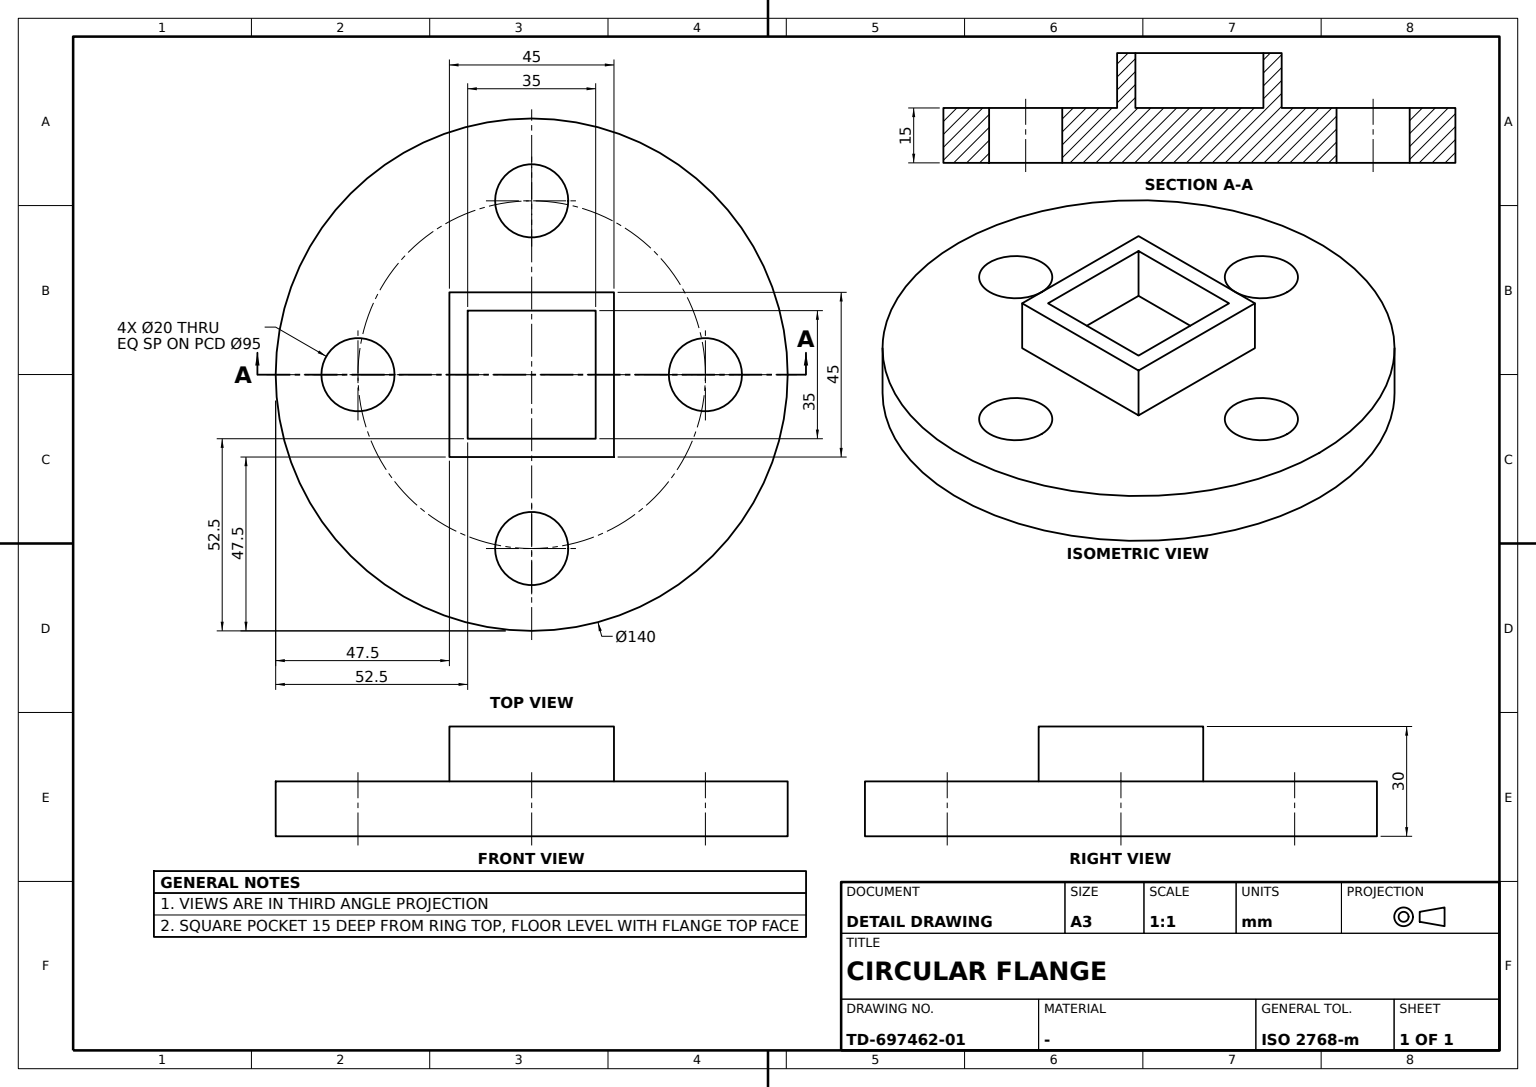
ISO-10303-21;
HEADER;
FILE_DESCRIPTION((''),'2;1');
FILE_NAME('','',(''),(''),'','','');
FILE_SCHEMA(('AUTOMOTIVE_DESIGN'));
ENDSEC;
DATA;
#1=APPLICATION_CONTEXT('');
#2=PRODUCT_CONTEXT('',#1,'mechanical');
#3=PRODUCT('','','',(#2));
#4=PRODUCT_DEFINITION_FORMATION('','',#3);
#5=PRODUCT_DEFINITION_CONTEXT('',#1,'design');
#6=PRODUCT_DEFINITION('','',#4,#5);
#7=PRODUCT_DEFINITION_SHAPE('','',#6);
#8=(LENGTH_UNIT()NAMED_UNIT(*)SI_UNIT(.MILLI.,.METRE.));
#9=(NAMED_UNIT(*)PLANE_ANGLE_UNIT()SI_UNIT($,.RADIAN.));
#10=(NAMED_UNIT(*)SI_UNIT($,.STERADIAN.)SOLID_ANGLE_UNIT());
#11=UNCERTAINTY_MEASURE_WITH_UNIT(LENGTH_MEASURE(0.005),#8,'distance_accuracy_value','');
#12=(GEOMETRIC_REPRESENTATION_CONTEXT(3)GLOBAL_UNCERTAINTY_ASSIGNED_CONTEXT((#11))GLOBAL_UNIT_ASSIGNED_CONTEXT((#8,#9,#10))REPRESENTATION_CONTEXT('',''));
#13=CARTESIAN_POINT('',(-17.5,-17.5,15.));
#14=VERTEX_POINT('',#13);
#15=CARTESIAN_POINT('',(-17.5,17.5,15.));
#16=VERTEX_POINT('',#15);
#17=CARTESIAN_POINT('',(-17.5,0.,15.));
#18=DIRECTION('',(0.,1.,0.));
#19=VECTOR('',#18,1000.);
#20=LINE('',#17,#19);
#21=EDGE_CURVE('',#14,#16,#20,.T.);
#22=ORIENTED_EDGE('',*,*,#21,.F.);
#23=CARTESIAN_POINT('',(17.5,-17.5,15.));
#24=VERTEX_POINT('',#23);
#25=CARTESIAN_POINT('',(0.,-17.5,15.));
#26=DIRECTION('',(-1.,0.,0.));
#27=VECTOR('',#26,1000.);
#28=LINE('',#25,#27);
#29=EDGE_CURVE('',#24,#14,#28,.T.);
#30=ORIENTED_EDGE('',*,*,#29,.F.);
#31=CARTESIAN_POINT('',(17.5,17.5,15.));
#32=VERTEX_POINT('',#31);
#33=CARTESIAN_POINT('',(17.5,0.,15.));
#34=DIRECTION('',(0.,-1.,0.));
#35=VECTOR('',#34,1000.);
#36=LINE('',#33,#35);
#37=EDGE_CURVE('',#32,#24,#36,.T.);
#38=ORIENTED_EDGE('',*,*,#37,.F.);
#39=CARTESIAN_POINT('',(0.,17.5,15.));
#40=DIRECTION('',(1.,0.,0.));
#41=VECTOR('',#40,1000.);
#42=LINE('',#39,#41);
#43=EDGE_CURVE('',#16,#32,#42,.T.);
#44=ORIENTED_EDGE('',*,*,#43,.F.);
#45=EDGE_LOOP('',(#22,#30,#38,#44));
#46=FACE_BOUND('',#45,.T.);
#47=CARTESIAN_POINT('',(0.,0.,15.));
#48=DIRECTION('',(0.,0.,1.));
#49=AXIS2_PLACEMENT_3D('',#47,#48,#40);
#50=PLANE('',#49);
#51=ADVANCED_FACE('',(#46),#50,.T.);
#52=CARTESIAN_POINT('',(-22.5,22.5,15.));
#53=VERTEX_POINT('',#52);
#54=CARTESIAN_POINT('',(-22.5,22.5,30.));
#55=VERTEX_POINT('',#54);
#56=VECTOR('',#48,1000.);
#57=LINE('',#52,#56);
#58=EDGE_CURVE('',#53,#55,#57,.T.);
#59=ORIENTED_EDGE('',*,*,#58,.T.);
#60=CARTESIAN_POINT('',(22.5,22.5,30.));
#61=VERTEX_POINT('',#60);
#62=CARTESIAN_POINT('',(0.,22.5,30.));
#63=LINE('',#62,#41);
#64=EDGE_CURVE('',#55,#61,#63,.T.);
#65=ORIENTED_EDGE('',*,*,#64,.T.);
#66=CARTESIAN_POINT('',(22.5,22.5,15.));
#67=VERTEX_POINT('',#66);
#68=LINE('',#66,#56);
#69=EDGE_CURVE('',#67,#61,#68,.T.);
#70=ORIENTED_EDGE('',*,*,#69,.F.);
#71=CARTESIAN_POINT('',(0.,22.5,15.));
#72=LINE('',#71,#41);
#73=EDGE_CURVE('',#53,#67,#72,.T.);
#74=ORIENTED_EDGE('',*,*,#73,.F.);
#75=EDGE_LOOP('',(#59,#65,#70,#74));
#76=FACE_BOUND('',#75,.T.);
#77=AXIS2_PLACEMENT_3D('',#52,#34,#40);
#78=PLANE('',#77);
#79=ADVANCED_FACE('',(#76),#78,.F.);
#80=CARTESIAN_POINT('',(-37.5,0.,0.));
#81=VERTEX_POINT('',#80);
#82=CARTESIAN_POINT('',(-47.5,0.,0.));
#83=AXIS2_PLACEMENT_3D('',#82,#48,#40);
#84=CIRCLE('',#83,10.);
#85=EDGE_CURVE('',#81,#81,#84,.T.);
#86=ORIENTED_EDGE('',*,*,#85,.F.);
#87=EDGE_LOOP('',(#86));
#88=FACE_BOUND('',#87,.T.);
#89=CARTESIAN_POINT('',(-37.5,0.,15.));
#90=VERTEX_POINT('',#89);
#91=CARTESIAN_POINT('',(-47.5,0.,15.));
#92=AXIS2_PLACEMENT_3D('',#91,#48,#40);
#93=CIRCLE('',#92,10.);
#94=EDGE_CURVE('',#90,#90,#93,.T.);
#95=ORIENTED_EDGE('',*,*,#94,.T.);
#96=EDGE_LOOP('',(#95));
#97=FACE_BOUND('',#96,.T.);
#98=CARTESIAN_POINT('',(-47.5,0.,7.5));
#99=AXIS2_PLACEMENT_3D('',#98,#48,#40);
#100=CYLINDRICAL_SURFACE('',#99,10.);
#101=ADVANCED_FACE('',(#88,#97),#100,.F.);
#102=CARTESIAN_POINT('',(-17.5,17.5,30.));
#103=VERTEX_POINT('',#102);
#104=CARTESIAN_POINT('',(17.5,17.5,30.));
#105=VERTEX_POINT('',#104);
#106=CARTESIAN_POINT('',(0.,17.5,30.));
#107=LINE('',#106,#41);
#108=EDGE_CURVE('',#103,#105,#107,.T.);
#109=ORIENTED_EDGE('',*,*,#108,.T.);
#110=CARTESIAN_POINT('',(17.5,-17.5,30.));
#111=VERTEX_POINT('',#110);
#112=CARTESIAN_POINT('',(17.5,0.,30.));
#113=LINE('',#112,#35);
#114=EDGE_CURVE('',#105,#111,#113,.T.);
#115=ORIENTED_EDGE('',*,*,#114,.T.);
#116=CARTESIAN_POINT('',(-17.5,-17.5,30.));
#117=VERTEX_POINT('',#116);
#118=CARTESIAN_POINT('',(0.,-17.5,30.));
#119=LINE('',#118,#27);
#120=EDGE_CURVE('',#111,#117,#119,.T.);
#121=ORIENTED_EDGE('',*,*,#120,.T.);
#122=CARTESIAN_POINT('',(-17.5,0.,30.));
#123=LINE('',#122,#19);
#124=EDGE_CURVE('',#117,#103,#123,.T.);
#125=ORIENTED_EDGE('',*,*,#124,.T.);
#126=EDGE_LOOP('',(#109,#115,#121,#125));
#127=FACE_BOUND('',#126,.T.);
#128=CARTESIAN_POINT('',(22.5,-22.5,30.));
#129=VERTEX_POINT('',#128);
#130=CARTESIAN_POINT('',(-22.5,-22.5,30.));
#131=VERTEX_POINT('',#130);
#132=CARTESIAN_POINT('',(0.,-22.5,30.));
#133=LINE('',#132,#27);
#134=EDGE_CURVE('',#129,#131,#133,.T.);
#135=ORIENTED_EDGE('',*,*,#134,.F.);
#136=CARTESIAN_POINT('',(22.5,0.,30.));
#137=LINE('',#136,#35);
#138=EDGE_CURVE('',#61,#129,#137,.T.);
#139=ORIENTED_EDGE('',*,*,#138,.F.);
#140=ORIENTED_EDGE('',*,*,#64,.F.);
#141=CARTESIAN_POINT('',(-22.5,0.,30.));
#142=LINE('',#141,#19);
#143=EDGE_CURVE('',#131,#55,#142,.T.);
#144=ORIENTED_EDGE('',*,*,#143,.F.);
#145=EDGE_LOOP('',(#135,#139,#140,#144));
#146=FACE_BOUND('',#145,.T.);
#147=CARTESIAN_POINT('',(0.,0.,30.));
#148=AXIS2_PLACEMENT_3D('',#147,#48,#40);
#149=PLANE('',#148);
#150=ADVANCED_FACE('',(#127,#146),#149,.T.);
#151=CARTESIAN_POINT('',(70.,0.,15.));
#152=VERTEX_POINT('',#151);
#153=CIRCLE('',#49,70.);
#154=EDGE_CURVE('',#152,#152,#153,.T.);
#155=ORIENTED_EDGE('',*,*,#154,.T.);
#156=EDGE_LOOP('',(#155));
#157=FACE_BOUND('',#156,.T.);
#158=CARTESIAN_POINT('',(10.,-47.5,15.));
#159=VERTEX_POINT('',#158);
#160=CARTESIAN_POINT('',(0.,-47.5,15.));
#161=AXIS2_PLACEMENT_3D('',#160,#48,#40);
#162=CIRCLE('',#161,10.);
#163=EDGE_CURVE('',#159,#159,#162,.T.);
#164=ORIENTED_EDGE('',*,*,#163,.F.);
#165=EDGE_LOOP('',(#164));
#166=FACE_BOUND('',#165,.T.);
#167=ORIENTED_EDGE('',*,*,#73,.T.);
#168=CARTESIAN_POINT('',(22.5,-22.5,15.));
#169=VERTEX_POINT('',#168);
#170=CARTESIAN_POINT('',(22.5,0.,15.));
#171=LINE('',#170,#35);
#172=EDGE_CURVE('',#67,#169,#171,.T.);
#173=ORIENTED_EDGE('',*,*,#172,.T.);
#174=CARTESIAN_POINT('',(-22.5,-22.5,15.));
#175=VERTEX_POINT('',#174);
#176=CARTESIAN_POINT('',(0.,-22.5,15.));
#177=LINE('',#176,#27);
#178=EDGE_CURVE('',#169,#175,#177,.T.);
#179=ORIENTED_EDGE('',*,*,#178,.T.);
#180=CARTESIAN_POINT('',(-22.5,0.,15.));
#181=LINE('',#180,#19);
#182=EDGE_CURVE('',#175,#53,#181,.T.);
#183=ORIENTED_EDGE('',*,*,#182,.T.);
#184=EDGE_LOOP('',(#167,#173,#179,#183));
#185=FACE_BOUND('',#184,.T.);
#186=ORIENTED_EDGE('',*,*,#94,.F.);
#187=EDGE_LOOP('',(#186));
#188=FACE_BOUND('',#187,.T.);
#189=CARTESIAN_POINT('',(57.5,0.,15.));
#190=VERTEX_POINT('',#189);
#191=CARTESIAN_POINT('',(47.5,0.,15.));
#192=AXIS2_PLACEMENT_3D('',#191,#48,#40);
#193=CIRCLE('',#192,10.);
#194=EDGE_CURVE('',#190,#190,#193,.T.);
#195=ORIENTED_EDGE('',*,*,#194,.F.);
#196=EDGE_LOOP('',(#195));
#197=FACE_BOUND('',#196,.T.);
#198=CARTESIAN_POINT('',(10.,47.5,15.));
#199=VERTEX_POINT('',#198);
#200=CARTESIAN_POINT('',(0.,47.5,15.));
#201=AXIS2_PLACEMENT_3D('',#200,#48,#40);
#202=CIRCLE('',#201,10.);
#203=EDGE_CURVE('',#199,#199,#202,.T.);
#204=ORIENTED_EDGE('',*,*,#203,.F.);
#205=EDGE_LOOP('',(#204));
#206=FACE_BOUND('',#205,.T.);
#207=ADVANCED_FACE('',(#157,#166,#185,#188,#197,#206),#50,.T.);
#208=ORIENTED_EDGE('',*,*,#163,.T.);
#209=EDGE_LOOP('',(#208));
#210=FACE_BOUND('',#209,.T.);
#211=CARTESIAN_POINT('',(10.,-47.5,0.));
#212=VERTEX_POINT('',#211);
#213=CARTESIAN_POINT('',(0.,-47.5,0.));
#214=AXIS2_PLACEMENT_3D('',#213,#48,#40);
#215=CIRCLE('',#214,10.);
#216=EDGE_CURVE('',#212,#212,#215,.T.);
#217=ORIENTED_EDGE('',*,*,#216,.F.);
#218=EDGE_LOOP('',(#217));
#219=FACE_BOUND('',#218,.T.);
#220=CARTESIAN_POINT('',(0.,-47.5,7.5));
#221=AXIS2_PLACEMENT_3D('',#220,#48,#40);
#222=CYLINDRICAL_SURFACE('',#221,10.);
#223=ADVANCED_FACE('',(#210,#219),#222,.F.);
#224=LINE('',#174,#56);
#225=EDGE_CURVE('',#175,#131,#224,.T.);
#226=ORIENTED_EDGE('',*,*,#225,.T.);
#227=ORIENTED_EDGE('',*,*,#143,.T.);
#228=ORIENTED_EDGE('',*,*,#58,.F.);
#229=ORIENTED_EDGE('',*,*,#182,.F.);
#230=EDGE_LOOP('',(#226,#227,#228,#229));
#231=FACE_BOUND('',#230,.T.);
#232=AXIS2_PLACEMENT_3D('',#174,#40,#18);
#233=PLANE('',#232);
#234=ADVANCED_FACE('',(#231),#233,.F.);
#235=ORIENTED_EDGE('',*,*,#114,.F.);
#236=LINE('',#31,#56);
#237=EDGE_CURVE('',#32,#105,#236,.T.);
#238=ORIENTED_EDGE('',*,*,#237,.F.);
#239=ORIENTED_EDGE('',*,*,#37,.T.);
#240=LINE('',#23,#56);
#241=EDGE_CURVE('',#24,#111,#240,.T.);
#242=ORIENTED_EDGE('',*,*,#241,.T.);
#243=EDGE_LOOP('',(#235,#238,#239,#242));
#244=FACE_BOUND('',#243,.T.);
#245=AXIS2_PLACEMENT_3D('',#31,#26,#34);
#246=PLANE('',#245);
#247=ADVANCED_FACE('',(#244),#246,.T.);
#248=CARTESIAN_POINT('',(10.,47.5,0.));
#249=VERTEX_POINT('',#248);
#250=CARTESIAN_POINT('',(0.,47.5,0.));
#251=AXIS2_PLACEMENT_3D('',#250,#48,#40);
#252=CIRCLE('',#251,10.);
#253=EDGE_CURVE('',#249,#249,#252,.T.);
#254=ORIENTED_EDGE('',*,*,#253,.F.);
#255=EDGE_LOOP('',(#254));
#256=FACE_BOUND('',#255,.T.);
#257=ORIENTED_EDGE('',*,*,#203,.T.);
#258=EDGE_LOOP('',(#257));
#259=FACE_BOUND('',#258,.T.);
#260=CARTESIAN_POINT('',(0.,47.5,7.5));
#261=AXIS2_PLACEMENT_3D('',#260,#48,#40);
#262=CYLINDRICAL_SURFACE('',#261,10.);
#263=ADVANCED_FACE('',(#256,#259),#262,.F.);
#264=ORIENTED_EDGE('',*,*,#194,.T.);
#265=EDGE_LOOP('',(#264));
#266=FACE_BOUND('',#265,.T.);
#267=CARTESIAN_POINT('',(57.5,0.,0.));
#268=VERTEX_POINT('',#267);
#269=CARTESIAN_POINT('',(47.5,0.,0.));
#270=AXIS2_PLACEMENT_3D('',#269,#48,#40);
#271=CIRCLE('',#270,10.);
#272=EDGE_CURVE('',#268,#268,#271,.T.);
#273=ORIENTED_EDGE('',*,*,#272,.F.);
#274=EDGE_LOOP('',(#273));
#275=FACE_BOUND('',#274,.T.);
#276=CARTESIAN_POINT('',(47.5,0.,7.5));
#277=AXIS2_PLACEMENT_3D('',#276,#48,#40);
#278=CYLINDRICAL_SURFACE('',#277,10.);
#279=ADVANCED_FACE('',(#266,#275),#278,.F.);
#280=ORIENTED_EDGE('',*,*,#108,.F.);
#281=LINE('',#15,#56);
#282=EDGE_CURVE('',#16,#103,#281,.T.);
#283=ORIENTED_EDGE('',*,*,#282,.F.);
#284=ORIENTED_EDGE('',*,*,#43,.T.);
#285=ORIENTED_EDGE('',*,*,#237,.T.);
#286=EDGE_LOOP('',(#280,#283,#284,#285));
#287=FACE_BOUND('',#286,.T.);
#288=AXIS2_PLACEMENT_3D('',#15,#34,#40);
#289=PLANE('',#288);
#290=ADVANCED_FACE('',(#287),#289,.T.);
#291=ORIENTED_EDGE('',*,*,#225,.F.);
#292=ORIENTED_EDGE('',*,*,#178,.F.);
#293=LINE('',#168,#56);
#294=EDGE_CURVE('',#169,#129,#293,.T.);
#295=ORIENTED_EDGE('',*,*,#294,.T.);
#296=ORIENTED_EDGE('',*,*,#134,.T.);
#297=EDGE_LOOP('',(#291,#292,#295,#296));
#298=FACE_BOUND('',#297,.T.);
#299=AXIS2_PLACEMENT_3D('',#168,#18,#26);
#300=PLANE('',#299);
#301=ADVANCED_FACE('',(#298),#300,.F.);
#302=ORIENTED_EDGE('',*,*,#120,.F.);
#303=ORIENTED_EDGE('',*,*,#241,.F.);
#304=ORIENTED_EDGE('',*,*,#29,.T.);
#305=LINE('',#13,#56);
#306=EDGE_CURVE('',#14,#117,#305,.T.);
#307=ORIENTED_EDGE('',*,*,#306,.T.);
#308=EDGE_LOOP('',(#302,#303,#304,#307));
#309=FACE_BOUND('',#308,.T.);
#310=AXIS2_PLACEMENT_3D('',#23,#18,#26);
#311=PLANE('',#310);
#312=ADVANCED_FACE('',(#309),#311,.T.);
#313=ORIENTED_EDGE('',*,*,#282,.T.);
#314=ORIENTED_EDGE('',*,*,#124,.F.);
#315=ORIENTED_EDGE('',*,*,#306,.F.);
#316=ORIENTED_EDGE('',*,*,#21,.T.);
#317=EDGE_LOOP('',(#313,#314,#315,#316));
#318=FACE_BOUND('',#317,.T.);
#319=AXIS2_PLACEMENT_3D('',#13,#40,#18);
#320=PLANE('',#319);
#321=ADVANCED_FACE('',(#318),#320,.T.);
#322=ORIENTED_EDGE('',*,*,#272,.T.);
#323=EDGE_LOOP('',(#322));
#324=FACE_BOUND('',#323,.T.);
#325=ORIENTED_EDGE('',*,*,#216,.T.);
#326=EDGE_LOOP('',(#325));
#327=FACE_BOUND('',#326,.T.);
#328=ORIENTED_EDGE('',*,*,#85,.T.);
#329=EDGE_LOOP('',(#328));
#330=FACE_BOUND('',#329,.T.);
#331=CARTESIAN_POINT('',(70.,0.,0.));
#332=VERTEX_POINT('',#331);
#333=CARTESIAN_POINT('',(0.,0.,0.));
#334=AXIS2_PLACEMENT_3D('',#333,#48,#40);
#335=CIRCLE('',#334,70.);
#336=EDGE_CURVE('',#332,#332,#335,.T.);
#337=ORIENTED_EDGE('',*,*,#336,.F.);
#338=EDGE_LOOP('',(#337));
#339=FACE_BOUND('',#338,.T.);
#340=ORIENTED_EDGE('',*,*,#253,.T.);
#341=EDGE_LOOP('',(#340));
#342=FACE_BOUND('',#341,.T.);
#343=PLANE('',#334);
#344=ADVANCED_FACE('',(#324,#327,#330,#339,#342),#343,.F.);
#345=ORIENTED_EDGE('',*,*,#336,.T.);
#346=EDGE_LOOP('',(#345));
#347=FACE_BOUND('',#346,.T.);
#348=ORIENTED_EDGE('',*,*,#154,.F.);
#349=EDGE_LOOP('',(#348));
#350=FACE_BOUND('',#349,.T.);
#351=CARTESIAN_POINT('',(0.,0.,7.5));
#352=AXIS2_PLACEMENT_3D('',#351,#48,#40);
#353=CYLINDRICAL_SURFACE('',#352,70.);
#354=ADVANCED_FACE('',(#347,#350),#353,.T.);
#355=ORIENTED_EDGE('',*,*,#172,.F.);
#356=ORIENTED_EDGE('',*,*,#69,.T.);
#357=ORIENTED_EDGE('',*,*,#138,.T.);
#358=ORIENTED_EDGE('',*,*,#294,.F.);
#359=EDGE_LOOP('',(#355,#356,#357,#358));
#360=FACE_BOUND('',#359,.T.);
#361=AXIS2_PLACEMENT_3D('',#66,#26,#34);
#362=PLANE('',#361);
#363=ADVANCED_FACE('',(#360),#362,.F.);
#364=CLOSED_SHELL('',(#51,#79,#101,#150,#207,#223,#234,#247,#263,#279,#290,#301,#312,#321,#344,#354,#363));
#365=MANIFOLD_SOLID_BREP('',#364);
#366=ADVANCED_BREP_SHAPE_REPRESENTATION('',(#365),#12);
#367=SHAPE_DEFINITION_REPRESENTATION(#7,#366);
ENDSEC;
END-ISO-10303-21;
